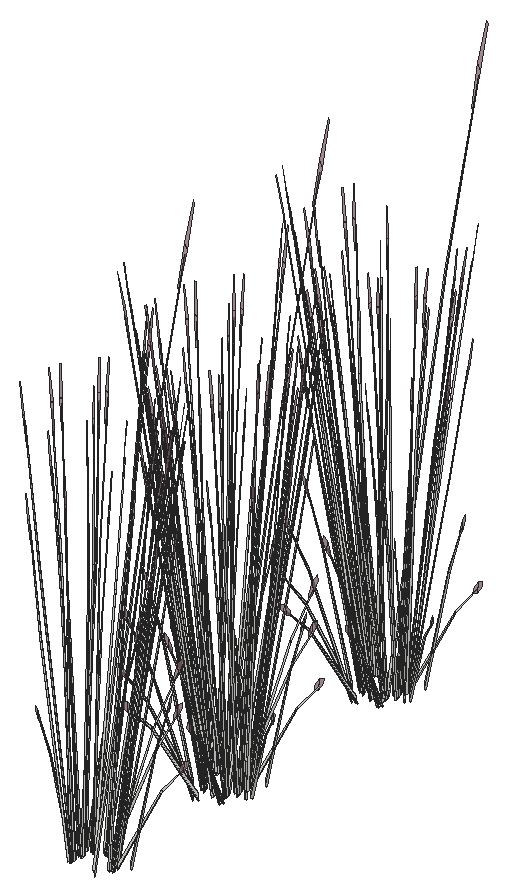
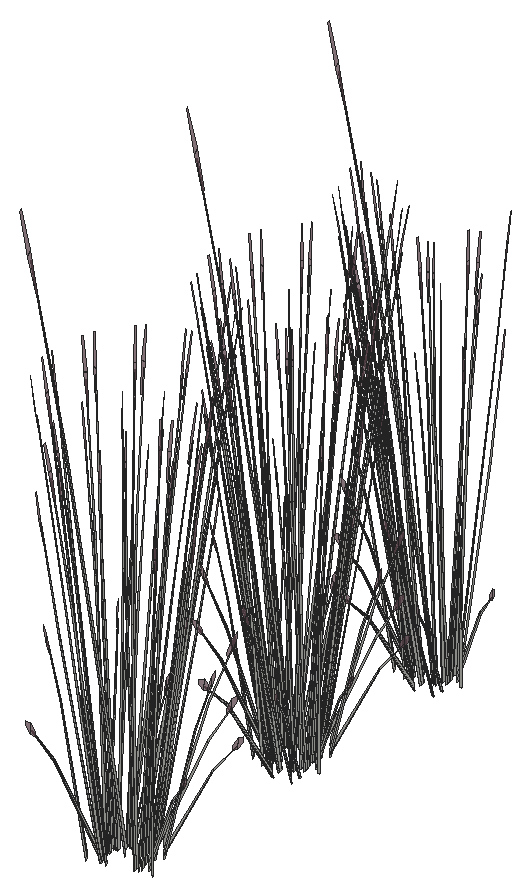
# SketchUp Ruby script. Lengths in inches.
U = 1.inch
M = Sketchup.active_model
def pt(a) = Geom::Point3d.new(a.map { |v| v * U })
def face(e, loops, mat)
  f = e.add_face(loops[0].map { |a| pt(a) })
  loops[1..].each { |l| e.add_face(l.map { |a| pt(a) }).erase! }
  f.material = f.back_material = mat if mat
  f
end
# faces: each face lists its corners as indices into pts; further lists are holes
def faces(e, pts, list, mat = nil) = list.each { |f| face(e, (f[0].is_a?(Array) ? f : [f]).map { |l| l.map { |i| pts[i] } }, mat) }
# xy, xz, yz: faces in a plane at the given z, y or x. An outline is a flat list of corners, or four numbers for a rectangle; further outlines are holes
def ring(l) = l.size == 4 ? [[l[0], l[1]], [l[2], l[1]], [l[2], l[3]], [l[0], l[3]]] : l.each_slice(2).to_a
def flat(e, list, mat, &to3) = list.each { |f| face(e, (f[0].is_a?(Array) ? f : [f]).map { |l| ring(l).map { |u, v| to3.(u, v) } }, mat) }
def xy(e, z, list, mat = nil) = flat(e, list, mat) { |x, y| [x, y, z] }
def xz(e, y, list, mat = nil) = flat(e, list, mat) { |x, z| [x, y, z] }
def yz(e, x, list, mat = nil) = flat(e, list, mat) { |y, z| [x, y, z] }
def lines(e, pts, list) = list.each { |a, b| e.add_line(pt(pts[a]), pt(pts[b])) }
# prism: a flat outline (further loops are holes) pulled along v
def prism(e, loops, v, mat = nil)
  f = face(e, loops, mat); d = Geom::Vector3d.new(v.map { |x| x * U })
  f.pushpull(f.normal.samedirection?(d) ? d.length : -d.length)
end
def box(e, o, s, mat = nil) = prism(e, [[o, [o[0] + s[0], o[1], o[2]], [o[0] + s[0], o[1] + s[1], o[2]], [o[0], o[1] + s[1], o[2]]]], [0, 0, s[2]], mat)
def at(x, y, z, deg = 0) = Geom::Transformation.translation(pt([x, y, z])) * Geom::Transformation.rotation(ORIGIN, Z_AXIS, deg.degrees)
def axes(o, x, y, z) = Geom::Transformation.new([*x, 0, *y, 0, *z, 0, *pt(o).to_a, 1])
def part(name) = M.definitions.add(name)
# library, detail: a bought-in or finely detailed component or shape, given as its bounding box
def library(name, o, s) = part(name).tap { |d| box(d.entities, o, s) }
def detail(e, o, s) = box(e.add_group.entities, o, s)
def put(e, d, t, mat = nil) = e.add_instance(d, t).tap { |i| i.material = mat if mat }
def group(e, t, mat = nil) = e.add_group.tap { |g| g.transformation = t; g.material = mat if mat }.entities
root = M.entities
M.materials.add("LightPink_Translucent").color = [144, 107, 117]
M.materials["LightPink_Translucent"].alpha = 0.75
c1 = part("blade")
p = [[2.15,0.21,22],[0,0.17,0],[0.09,0.45,0],[2.18,0.31,22],[2.29,0.31,22],[0.38,0.45,0],
  [2.48,0.24,33],[2.49,0.24,33],[2.48,0.22,33]]
faces(c1.entities,p,[[0,1,2,3],[4,5,2,3],[6,3,4,7],[8,0,3,6]])
c2 = part("seeds")
p = [[0.3,-0.1,1.38],[-0.01,-0.03,1.59],[-0.01,-0.03,0.03],[0.14,-0.07,-0.07],[0.29,-0.03,3],[0.15,0.01,3.11]]
faces(c2.entities,p,[[0,1,2,3],[1,0,4,5]],"LightPink_Translucent")
c3 = part("blade with seeds")
put(c3.entities,c1,at(0,0,0))
put(c3.entities,c2,axes([2.4,0.25,30.99],[1.5799,-0.05474,1.17369],[-0.12525,1.92788,0.29478],[-0.07173,-0.02425,1.56792]))
put(root,c3,axes([403.47,675.8,5.05],[-0.29332,-0.1301,0.35414],[0.08555,-0.37955,-0.4572],[0.11809,-0.0348,0.87481]))
put(root,c3,axes([400.4,675.11,4.73],[0.09971,-0.42522,0.48003],[0.32782,0.1454,0.3958],[-0.12892,0.02555,0.9933]))
put(root,c3,axes([400.37,675,4.73],[-0.12963,-0.31798,0.0643],[0.23638,-0.15564,0.50621],[-0.1042,0.03071,0.77189]))
put(root,c3,axes([403.73,675.92,4.73],[0.12963,0.31798,0.0643],[-0.23638,0.15564,0.50621],[0.1042,-0.03071,0.77189]))
put(root,c3,axes([403.71,675.81,4.73],[-0.09971,0.42522,0.48003],[-0.32782,-0.1454,0.3958],[0.12892,-0.02555,0.9933]))
put(root,c3,axes([400.64,675.12,5.05],[0.29332,0.1301,0.35414],[-0.08555,0.37955,-0.4572],[-0.11809,0.0348,0.87481]))
put(root,c3,axes([404.3,677.1875,4.71],[-0.03191,-0.04083,1.77383],[0.06981,-0.43764,-0.16761],[0.12571,-0.02796,0.31391]))
put(root,c3,axes([400.14,675.41,4.72],[-0.05763,0.06055,1.74944],[0.0049,0.44239,-0.27667],[-0.13211,0.05753,0.14031]))
put(root,c3,axes([400.51,674.99,5.03],[0.17758,0.42229,-0.1216],[-0.31518,0.20752,-0.67495],[-0.13282,0.05572,1.02557]))
put(root,c3,axes([403.19,676.81,5.03],[0.0189,-0.47427,-0.1216],[0.35781,0.01296,-0.67495],[0.13781,0.03295,1.02557]))
put(root,c3,axes([403.14,676.62,5.05],[-0.20082,-0.29199,0.35414],[0.2293,-0.2764,-0.4572],[0.1165,0.04206,0.87481]))
put(root,c3,axes([403.5,676.52,4.72],[0.07571,-0.00789,1.74944],[0.20767,-0.36231,-0.27667],[0.13467,0.04783,0.14031]))
put(root,c3,axes([400.47,676.17,4.73],[-0.08753,-0.42921,0.48003],[0.34336,-0.07449,0.3958],[-0.1012,0.10094,0.9933]))
put(root,c3,axes([400.41,676.09,4.73],[-0.2423,-0.19613,0.0643],[0.14107,-0.2793,0.50621],[-0.07768,0.0903,0.77189]))
put(root,c3,axes([400.6875,676.03,5.05],[0.30722,-0.06665,0.35414],[0.08112,0.381,-0.4572],[-0.08804,0.10234,0.87481]))
put(root,c3,axes([399.5,675.86,4.71],[0.04504,0.01251,1.77383],[0.13934,0.41205,-0.16761],[-0.0922,0.10815,0.31391]))
put(root,c3,axes([403.32,676.89,4.73],[-0.01777,0.35463,0.0643],[-0.26836,-0.00972,0.50621],[0.1028,0.03711,0.77189]))
put(root,c3,axes([403.34,676.77,4.73],[-0.26024,0.30729,0.48003],[-0.22444,-0.32634,0.3958],[0.1221,0.05668,0.9933]))
put(root,c3,axes([399.99,677.11,5.65],[0.31145,0.12449,-0.06488],[-0.0958,0.38314,-0.29416],[-0.05094,0.05817,0.97024]))
put(root,c3,axes([402.52,677.13,5.05],[-0.05451,-0.37564,0.35414],[0.31161,-0.09919,-0.4572],[0.0837,0.10765,0.87481]))
put(root,c3,axes([402.72,674.97,4.47],[-0.30498,-0.24231,1.38283],[0.32203,-0.37727,0.59665],[0.0984,0.22736,1.33663]))
put(root,c3,axes([400.53,675.99,5.03],[0.32648,0.25715,-0.1216],[-0.18809,0.3724,-0.67495],[-0.09224,0.12945,1.02557]))
put(root,c3,axes([402.49,677.32,5.03],[0.21031,-0.39918,-0.1216],[0.30457,0.22997,-0.67495],[0.10587,0.11278,1.02557]))
put(root,c3,axes([401.1,676.79,5.05],[0.23881,-0.24554,0.35414],[0.22606,0.28036,-0.4572],[-0.0344,0.14245,0.87481]))
put(root,c3,axes([402.21,677.66,4.71],[0.00104,-0.05646,1.77383],[0.30246,-0.2491,-0.16761],[0.10506,0.08891,0.31391]))
put(root,c3,axes([400.88,677.01,4.73],[-0.29004,-0.02173,0.0643],[0.00795,-0.32812,0.50621],[-0.03035,0.12569,0.77189]))
put(root,c3,axes([400.98,677.04,4.73],[-0.25132,-0.3182,0.48003],[0.2669,-0.27442,0.3958],[-0.04636,0.14929,0.9933]))
put(root,c3,axes([401.77,677.19,5.05],[0.1064,-0.35863,0.35414],[0.31043,0.1046,-0.4572],[0.02846,0.14439,0.87481]))
put(root,c3,axes([402.56,677.47,4.73],[-0.16041,0.29625,0.0643],[-0.22843,-0.17248,0.50621],[0.07385,0.09498,0.77189]))
put(root,c3,axes([402.1875,678.47,5.65],[0.2439,-0.26754,-0.06488],[0.22348,0.29302,-0.29416],[0.01573,0.08303,0.97024]))
put(root,c3,axes([402.63,677.39,4.73],[-0.35104,0.10702,0.48003],[-0.06092,-0.41983,0.3958],[0.08256,0.12373,0.9933]))
put(root,c3,axes([401.67,677.51,4.73],[-0.26007,0.1585,0.0643],[-0.12729,-0.28902,0.50621],[0.02512,0.1274,0.77189]))
put(root,c3,axes([400.15,677.0625,4.72],[-0.00877,0.09229,1.74944],[0.24897,0.32105,-0.27667],[-0.06518,0.15182,0.14031]))
put(root,c3,axes([400.95,676.85,5.4],[0.3879,0.02311,-0.13498],[-0.0106,0.43749,-0.74919],[-0.02694,0.1685,1.13838]))
put(root,c3,axes([401.67,677.34,5.03],[0.34538,-0.21713,-0.1216],[0.16972,0.38536,-0.67495],[0.04557,0.16239,1.02557]))
put(root,c3,axes([401.77,677.48,5.0625],[-0.34777,-0.12192,0.53283],[0.11892,-0.40083,0.43934],[0.0209,0.15763,1.10256]))
put(root,c3,axes([400.125,678.01,4.71],[0.04004,-0.02816,1.77383],[0.33095,0.18728,-0.16761],[-0.00778,0.15594,0.31391]))
put(root,c3,axes([401.58,678.2,4.72],[0.04474,0.0751,1.74944],[0.36104,0.0295,-0.27667],[0.03631,0.16562,0.14031]))
put(root,c3,axes([401.89,687.65,4.72],[-0.05398,-0.06539,1.74944],[-0.36026,0.04145,-0.27667],[-0.0575,-0.15639,0.14031]))
put(root,c3,axes([403.51,688.45,4.72],[-0.00341,-0.09282,1.74944],[-0.28775,-0.26825,-0.27667],[0.04449,-0.16261,0.14031]))
put(root,c3,axes([403.43,688.11,4.71],[-0.03584,0.03562,1.77383],[-0.35118,-0.12018,-0.16761],[-0.01271,-0.15545,0.31391]))
put(root,c3,axes([401.52,687.43,4.71],[-0.00658,0.0559,1.77383],[-0.32474,0.20287,-0.16761],[-0.09556,-0.1037,0.31391]))
put(root,c3,axes([401.45,688.42,5.09],[0.39316,-0.11987,0.53763],[0.06823,0.47021,0.4433],[-0.09247,-0.13858,1.11249]))
put(root,c3,axes([402.34,688.51,4.73],[0.34777,0.12192,0.48003],[-0.11892,0.40083,0.3958],[-0.0209,-0.15763,0.9933]))
put(root,c3,axes([402.4375,688.65,5.03],[-0.34538,0.21713,-0.1216],[-0.16972,-0.38536,-0.67495],[-0.04557,-0.16239,1.02557]))
put(root,c3,axes([403.15,689.14,5.03],[-0.3879,-0.02311,-0.1216],[0.0106,-0.43749,-0.67495],[0.02694,-0.1685,1.02557]))
put(root,c3,axes([402.43,688.48,4.73],[0.26007,-0.1585,0.0643],[0.12729,0.28902,0.50621],[-0.02512,-0.1274,0.77189]))
put(root,c3,axes([401.54,688.52,4.73],[0.16041,-0.29625,0.0643],[0.22843,0.17248,0.50621],[-0.07385,-0.09498,0.77189]))
put(root,c3,axes([402.33,688.81,5.05],[-0.1064,0.35863,0.35414],[-0.31043,-0.1046,-0.4572],[-0.02846,-0.14439,0.87481]))
put(root,c3,axes([403.125,688.96,4.73],[0.25132,0.3182,0.48003],[-0.2669,0.27442,0.3958],[0.04636,-0.14929,0.9933]))
put(root,c3,axes([401.61,688.49,5.43],[-0.23555,0.44708,-0.13619],[-0.34112,-0.25757,-0.75594],[-0.11858,-0.12631,1.14864]))
put(root,c3,axes([403.22,688.99,4.73],[0.29004,0.02173,0.0643],[-0.00795,0.32812,0.50621],[0.03035,-0.12569,0.77189]))
put(root,c3,axes([403,689.21,5.05],[-0.23881,0.24554,0.35414],[-0.22606,-0.28036,-0.4572],[0.0344,-0.14245,0.87481]))
put(root,c3,axes([400.71,688.36,4.72],[-0.07594,-0.00329,1.74944],[-0.24177,0.32918,-0.27667],[-0.129,-0.06726,0.14031]))
put(root,c3,axes([403.58,690,5.03],[-0.32648,-0.25715,-0.1216],[0.18809,-0.3724,-0.67495],[0.09224,-0.12945,1.02557]))
put(root,c3,axes([401.59,688.86,5.05],[0.05451,0.37564,0.35414],[-0.31161,0.09919,-0.4572],[-0.0837,-0.10765,0.87481]))
put(root,c3,axes([400.65,689.11,5.09],[0.29147,-0.34417,0.53763],[0.25138,0.3655,0.4433],[-0.13675,-0.06349,1.11249]))
put(root,c3,axes([404.38,689.89,4.71],[-0.0461,-0.00354,1.77383],[-0.19143,-0.37951,-0.16761],[0.07688,-0.12478,0.31391]))
put(root,c3,axes([400.78,689.11,4.73],[0.01777,-0.35463,0.0643],[0.26836,0.00972,0.50621],[-0.1028,-0.03711,0.77189]))
put(root,c3,axes([403.42,689.97,5.05],[-0.30722,0.06665,0.35414],[-0.08112,-0.381,-0.4572],[0.08804,-0.10234,0.87481]))
put(root,c3,axes([403.7,689.91,4.73],[0.2423,0.19613,0.0643],[-0.14107,0.2793,0.50621],[0.07768,-0.0903,0.77189]))
put(root,c3,axes([403.63,689.83,4.73],[0.08753,0.42921,0.48003],[-0.34336,0.07449,0.3958],[0.1012,-0.10094,0.9933]))
put(root,c3,axes([404.55,690.34,4.72],[0.04898,-0.07104,1.74944],[-0.06269,-0.43574,-0.27667],[0.12289,-0.08262,0.14031]))
put(root,c3,axes([400.42,688.64,4.71],[0.02617,0.04654,1.77383],[-0.12614,0.41836,-0.16761],[-0.12775,0.00303,0.31391]))
put(root,c3,axes([400.97,689.37,5.05],[0.20082,0.29199,0.35414],[-0.2293,0.2764,-0.4572],[-0.1165,-0.04206,0.87481]))
put(root,c3,axes([400.91,689.1875,5.03],[-0.0189,0.47427,-0.1216],[-0.35781,-0.01296,-0.67495],[-0.13781,-0.03295,1.02557]))
put(root,c3,axes([403.59,691.01,5.03],[-0.17758,-0.42229,-0.1216],[0.31518,-0.20752,-0.67495],[0.13282,-0.05572,1.02557]))
put(root,c3,axes([403.47,690.88,5.05],[-0.29332,-0.1301,0.35414],[0.08555,-0.37955,-0.4572],[0.11809,-0.0348,0.87481]))
put(root,c3,axes([400.4,690.1875,4.73],[0.09971,-0.42522,0.48003],[0.32782,0.1454,0.3958],[-0.12892,0.02555,0.9933]))
put(root,c3,axes([400.37,690.07,4.73],[-0.12963,-0.31798,0.0643],[0.23638,-0.15564,0.50621],[-0.1042,0.03071,0.77189]))
put(root,c3,axes([403.73,691,4.73],[0.12963,0.31798,0.0643],[-0.23638,0.15564,0.50621],[0.1042,-0.03071,0.77189]))
put(root,c3,axes([403.71,690.88,4.73],[-0.09971,0.42522,0.48003],[-0.32782,-0.1454,0.3958],[0.12892,-0.02555,0.9933]))
put(root,c3,axes([400.64,690.19,5.05],[0.29332,0.1301,0.35414],[-0.08555,0.37955,-0.4572],[-0.11809,0.0348,0.87481]))
put(root,c3,axes([404.3,692.26,4.71],[-0.03191,-0.04083,1.77383],[0.06981,-0.43764,-0.16761],[0.12571,-0.02796,0.31391]))
put(root,c3,axes([400.14,690.49,4.72],[-0.05763,0.06055,1.74944],[0.0049,0.44239,-0.27667],[-0.13211,0.05753,0.14031]))
put(root,c3,axes([400.51,690.0625,5.03],[0.17758,0.42229,-0.1216],[-0.31518,0.20752,-0.67495],[-0.13282,0.05572,1.02557]))
put(root,c3,axes([403.19,691.88,5.03],[0.0189,-0.47427,-0.1216],[0.35781,0.01296,-0.67495],[0.13781,0.03295,1.02557]))
put(root,c3,axes([403.14,691.7,5.05],[-0.20082,-0.29199,0.35414],[0.2293,-0.2764,-0.4572],[0.1165,0.04206,0.87481]))
put(root,c3,axes([403.5,691.6,4.72],[0.07571,-0.00789,1.74944],[0.20767,-0.36231,-0.27667],[0.13467,0.04783,0.14031]))
put(root,c3,axes([400.47,691.24,4.73],[-0.08753,-0.42921,0.48003],[0.34336,-0.07449,0.3958],[-0.1012,0.10094,0.9933]))
put(root,c3,axes([400.41,691.16,4.73],[-0.2423,-0.19613,0.0643],[0.14107,-0.2793,0.50621],[-0.07768,0.0903,0.77189]))
put(root,c3,axes([400.6875,691.1,5.05],[0.30722,-0.06665,0.35414],[0.08112,0.381,-0.4572],[-0.08804,0.10234,0.87481]))
put(root,c3,axes([399.5,690.93,4.71],[0.04504,0.01251,1.77383],[0.13934,0.41205,-0.16761],[-0.0922,0.10815,0.31391]))
put(root,c3,axes([403.32,691.96,4.73],[-0.01777,0.35463,0.0643],[-0.26836,-0.00972,0.50621],[0.1028,0.03711,0.77189]))
put(root,c3,axes([403.34,691.85,4.73],[-0.26024,0.30729,0.48003],[-0.22444,-0.32634,0.3958],[0.1221,0.05668,0.9933]))
put(root,c3,axes([399.99,692.18,5.65],[0.31145,0.12449,-0.06488],[-0.0958,0.38314,-0.29416],[-0.05094,0.05817,0.97024]))
put(root,c3,axes([402.52,692.21,5.05],[-0.05451,-0.37564,0.35414],[0.31161,-0.09919,-0.4572],[0.0837,0.10765,0.87481]))
put(root,c3,axes([402.72,690.04,4.47],[-0.30498,-0.24231,1.38283],[0.32203,-0.37727,0.59665],[0.0984,0.22736,1.33663]))
put(root,c3,axes([400.53,691.07,5.03],[0.32648,0.25715,-0.1216],[-0.18809,0.3724,-0.67495],[-0.09224,0.12945,1.02557]))
put(root,c3,axes([402.49,692.4,5.03],[0.21031,-0.39918,-0.1216],[0.30457,0.22997,-0.67495],[0.10587,0.11278,1.02557]))
put(root,c3,axes([401.1,691.86,5.05],[0.23881,-0.24554,0.35414],[0.22606,0.28036,-0.4572],[-0.0344,0.14245,0.87481]))
put(root,c3,axes([402.21,692.73,4.71],[0.00104,-0.05646,1.77383],[0.30246,-0.2491,-0.16761],[0.10506,0.08891,0.31391]))
put(root,c3,axes([400.88,692.08,4.73],[-0.29004,-0.02173,0.0643],[0.00795,-0.32812,0.50621],[-0.03035,0.12569,0.77189]))
put(root,c3,axes([400.98,692.11,4.73],[-0.25132,-0.3182,0.48003],[0.2669,-0.27442,0.3958],[-0.04636,0.14929,0.9933]))
put(root,c3,axes([401.77,692.26,5.05],[0.1064,-0.35863,0.35414],[0.31043,0.1046,-0.4572],[0.02846,0.14439,0.87481]))
put(root,c3,axes([402.56,692.55,4.73],[-0.16041,0.29625,0.0643],[-0.22843,-0.17248,0.50621],[0.07385,0.09498,0.77189]))
put(root,c3,axes([402.1875,693.54,5.65],[0.2439,-0.26754,-0.06488],[0.22348,0.29302,-0.29416],[0.01573,0.08303,0.97024]))
put(root,c3,axes([402.63,692.46,4.73],[-0.35104,0.10702,0.48003],[-0.06092,-0.41983,0.3958],[0.08256,0.12373,0.9933]))
put(root,c3,axes([401.67,692.59,4.73],[-0.26007,0.1585,0.0643],[-0.12729,-0.28902,0.50621],[0.02512,0.1274,0.77189]))
put(root,c3,axes([400.15,692.14,4.72],[-0.00877,0.09229,1.74944],[0.24897,0.32105,-0.27667],[-0.06518,0.15182,0.14031]))
put(root,c3,axes([400.95,691.93,5.4],[0.3879,0.02311,-0.13498],[-0.0106,0.43749,-0.74919],[-0.02694,0.1685,1.13838]))
put(root,c3,axes([401.67,692.42,5.03],[0.34538,-0.21713,-0.1216],[0.16972,0.38536,-0.67495],[0.04557,0.16239,1.02557]))
put(root,c3,axes([401.77,692.56,5.0625],[-0.34777,-0.12192,0.53283],[0.11892,-0.40083,0.43934],[0.0209,0.15763,1.10256]))
put(root,c3,axes([400.125,693.08,4.71],[0.04004,-0.02816,1.77383],[0.33095,0.18728,-0.16761],[-0.00778,0.15594,0.31391]))
put(root,c3,axes([401.58,693.28,4.72],[0.04474,0.0751,1.74944],[0.36104,0.0295,-0.27667],[0.03631,0.16562,0.14031]))
put(root,c3,axes([401.89,705.37,4.72],[-0.05398,-0.06539,1.74944],[-0.36026,0.04145,-0.27667],[-0.0575,-0.15639,0.14031]))
put(root,c3,axes([403.51,706.17,4.72],[-0.00341,-0.09282,1.74944],[-0.28775,-0.26825,-0.27667],[0.04449,-0.16261,0.14031]))
put(root,c3,axes([403.43,705.84,4.71],[-0.03584,0.03562,1.77383],[-0.35118,-0.12018,-0.16761],[-0.01271,-0.15545,0.31391]))
put(root,c3,axes([401.52,705.16,4.71],[-0.00658,0.0559,1.77383],[-0.32474,0.20287,-0.16761],[-0.09556,-0.1037,0.31391]))
put(root,c3,axes([401.45,706.15,5.09],[0.39316,-0.11987,0.53763],[0.06823,0.47021,0.4433],[-0.09247,-0.13858,1.11249]))
put(root,c3,axes([402.34,706.24,4.73],[0.34777,0.12192,0.48003],[-0.11892,0.40083,0.3958],[-0.0209,-0.15763,0.9933]))
put(root,c3,axes([402.4375,706.38,5.03],[-0.34538,0.21713,-0.1216],[-0.16972,-0.38536,-0.67495],[-0.04557,-0.16239,1.02557]))
put(root,c3,axes([403.15,706.87,5.03],[-0.3879,-0.02311,-0.1216],[0.0106,-0.43749,-0.67495],[0.02694,-0.1685,1.02557]))
put(root,c3,axes([402.43,706.21,4.73],[0.26007,-0.1585,0.0643],[0.12729,0.28902,0.50621],[-0.02512,-0.1274,0.77189]))
put(root,c3,axes([401.54,706.25,4.73],[0.16041,-0.29625,0.0643],[0.22843,0.17248,0.50621],[-0.07385,-0.09498,0.77189]))
put(root,c3,axes([402.33,706.53,5.05],[-0.1064,0.35863,0.35414],[-0.31043,-0.1046,-0.4572],[-0.02846,-0.14439,0.87481]))
put(root,c3,axes([403.125,706.68,4.73],[0.25132,0.3182,0.48003],[-0.2669,0.27442,0.3958],[0.04636,-0.14929,0.9933]))
put(root,c3,axes([401.61,706.22,5.43],[-0.23555,0.44708,-0.13619],[-0.34112,-0.25757,-0.75594],[-0.11858,-0.12631,1.14864]))
put(root,c3,axes([403.22,706.71,4.73],[0.29004,0.02173,0.0643],[-0.00795,0.32812,0.50621],[0.03035,-0.12569,0.77189]))
put(root,c3,axes([403,706.9375,5.05],[-0.23881,0.24554,0.35414],[-0.22606,-0.28036,-0.4572],[0.0344,-0.14245,0.87481]))
put(root,c3,axes([400.71,706.09,4.72],[-0.07594,-0.00329,1.74944],[-0.24177,0.32918,-0.27667],[-0.129,-0.06726,0.14031]))
put(root,c3,axes([403.58,707.73,5.03],[-0.32648,-0.25715,-0.1216],[0.18809,-0.3724,-0.67495],[0.09224,-0.12945,1.02557]))
put(root,c3,axes([401.59,706.59,5.05],[0.05451,0.37564,0.35414],[-0.31161,0.09919,-0.4572],[-0.0837,-0.10765,0.87481]))
put(root,c3,axes([400.65,706.84,5.09],[0.29147,-0.34417,0.53763],[0.25138,0.3655,0.4433],[-0.13675,-0.06349,1.11249]))
put(root,c3,axes([404.38,707.62,4.71],[-0.0461,-0.00354,1.77383],[-0.19143,-0.37951,-0.16761],[0.07688,-0.12478,0.31391]))
put(root,c3,axes([400.78,706.83,4.73],[0.01777,-0.35463,0.0643],[0.26836,0.00972,0.50621],[-0.1028,-0.03711,0.77189]))
put(root,c3,axes([403.42,707.7,5.05],[-0.30722,0.06665,0.35414],[-0.08112,-0.381,-0.4572],[0.08804,-0.10234,0.87481]))
put(root,c3,axes([403.7,707.64,4.73],[0.2423,0.19613,0.0643],[-0.14107,0.2793,0.50621],[0.07768,-0.0903,0.77189]))
put(root,c3,axes([403.63,707.55,4.73],[0.08753,0.42921,0.48003],[-0.34336,0.07449,0.3958],[0.1012,-0.10094,0.9933]))
put(root,c3,axes([404.55,708.07,4.72],[0.04898,-0.07104,1.74944],[-0.06269,-0.43574,-0.27667],[0.12289,-0.08262,0.14031]))
put(root,c3,axes([400.42,706.37,4.71],[0.02617,0.04654,1.77383],[-0.12614,0.41836,-0.16761],[-0.12775,0.00303,0.31391]))
put(root,c3,axes([400.97,707.1,5.05],[0.20082,0.29199,0.35414],[-0.2293,0.2764,-0.4572],[-0.1165,-0.04206,0.87481]))
put(root,c3,axes([400.91,706.91,5.03],[-0.0189,0.47427,-0.1216],[-0.35781,-0.01296,-0.67495],[-0.13781,-0.03295,1.02557]))
put(root,c3,axes([403.59,708.73,5.03],[-0.17758,-0.42229,-0.1216],[0.31518,-0.20752,-0.67495],[0.13282,-0.05572,1.02557]))
put(root,c3,axes([403.47,708.61,5.05],[-0.29332,-0.1301,0.35414],[0.08555,-0.37955,-0.4572],[0.11809,-0.0348,0.87481]))
put(root,c3,axes([400.4,707.91,4.73],[0.09971,-0.42522,0.48003],[0.32782,0.1454,0.3958],[-0.12892,0.02555,0.9933]))
put(root,c3,axes([400.37,707.8,4.73],[-0.12963,-0.31798,0.0643],[0.23638,-0.15564,0.50621],[-0.1042,0.03071,0.77189]))
put(root,c3,axes([403.73,708.72,4.73],[0.12963,0.31798,0.0643],[-0.23638,0.15564,0.50621],[0.1042,-0.03071,0.77189]))
put(root,c3,axes([403.71,708.61,4.73],[-0.09971,0.42522,0.48003],[-0.32782,-0.1454,0.3958],[0.12892,-0.02555,0.9933]))
put(root,c3,axes([400.64,707.92,5.05],[0.29332,0.1301,0.35414],[-0.08555,0.37955,-0.4572],[-0.11809,0.0348,0.87481]))
put(root,c3,axes([404.3,709.99,4.71],[-0.03191,-0.04083,1.77383],[0.06981,-0.43764,-0.16761],[0.12571,-0.02796,0.31391]))
put(root,c3,axes([400.14,708.21,4.72],[-0.05763,0.06055,1.74944],[0.0049,0.44239,-0.27667],[-0.13211,0.05753,0.14031]))
put(root,c3,axes([400.51,707.79,5.03],[0.17758,0.42229,-0.1216],[-0.31518,0.20752,-0.67495],[-0.13282,0.05572,1.02557]))
put(root,c3,axes([403.19,709.61,5.03],[0.0189,-0.47427,-0.1216],[0.35781,0.01296,-0.67495],[0.13781,0.03295,1.02557]))
put(root,c3,axes([403.14,709.43,5.05],[-0.20082,-0.29199,0.35414],[0.2293,-0.2764,-0.4572],[0.1165,0.04206,0.87481]))
put(root,c3,axes([403.5,709.33,4.72],[0.07571,-0.00789,1.74944],[0.20767,-0.36231,-0.27667],[0.13467,0.04783,0.14031]))
put(root,c3,axes([400.47,708.97,4.73],[-0.08753,-0.42921,0.48003],[0.34336,-0.07449,0.3958],[-0.1012,0.10094,0.9933]))
put(root,c3,axes([400.41,708.89,4.73],[-0.2423,-0.19613,0.0643],[0.14107,-0.2793,0.50621],[-0.07768,0.0903,0.77189]))
put(root,c3,axes([400.6875,708.83,5.05],[0.30722,-0.06665,0.35414],[0.08112,0.381,-0.4572],[-0.08804,0.10234,0.87481]))
put(root,c3,axes([399.5,708.66,4.71],[0.04504,0.01251,1.77383],[0.13934,0.41205,-0.16761],[-0.0922,0.10815,0.31391]))
put(root,c3,axes([403.32,709.69,4.73],[-0.01777,0.35463,0.0643],[-0.26836,-0.00972,0.50621],[0.1028,0.03711,0.77189]))
put(root,c3,axes([403.34,709.58,4.73],[-0.26024,0.30729,0.48003],[-0.22444,-0.32634,0.3958],[0.1221,0.05668,0.9933]))
put(root,c3,axes([399.99,709.91,5.65],[0.31145,0.12449,-0.06488],[-0.0958,0.38314,-0.29416],[-0.05094,0.05817,0.97024]))
put(root,c3,axes([402.52,709.93,5.05],[-0.05451,-0.37564,0.35414],[0.31161,-0.09919,-0.4572],[0.0837,0.10765,0.87481]))
put(root,c3,axes([402.72,707.77,4.47],[-0.30498,-0.24231,1.38283],[0.32203,-0.37727,0.59665],[0.0984,0.22736,1.33663]))
